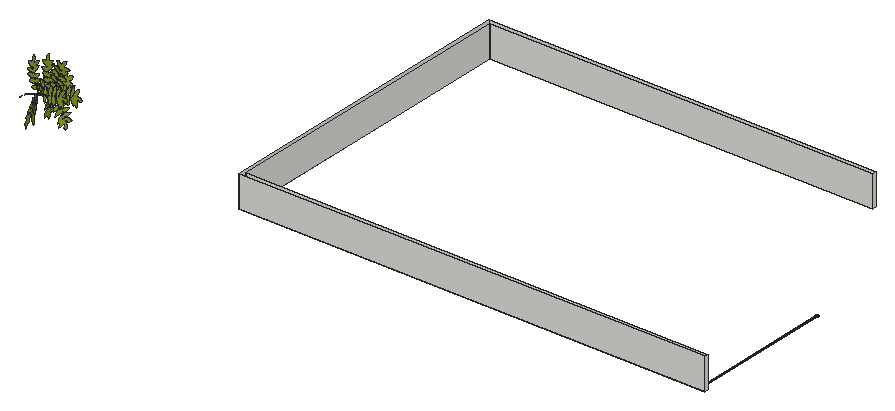
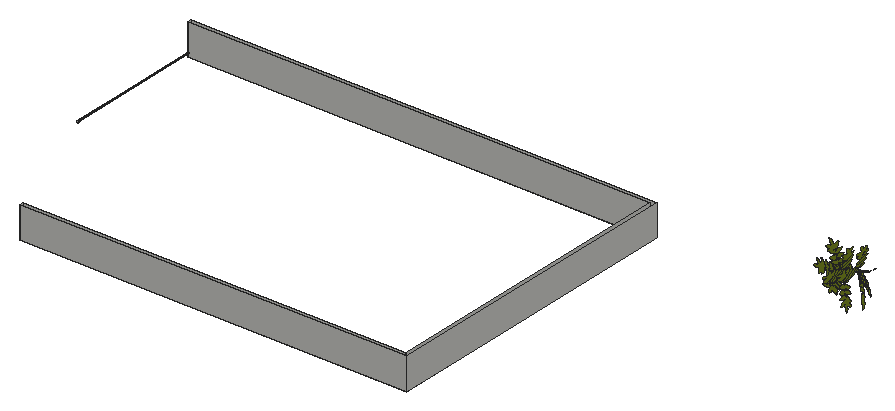
# SketchUp Ruby script. Lengths in inches.
U = 1.inch
M = Sketchup.active_model
def pt(a) = Geom::Point3d.new(a.map { |v| v * U })
def face(e, loops, mat)
  f = e.add_face(loops[0].map { |a| pt(a) })
  loops[1..].each { |l| e.add_face(l.map { |a| pt(a) }).erase! }
  f.material = f.back_material = mat if mat
  f
end
# faces: each face lists its corners as indices into pts; further lists are holes
def faces(e, pts, list, mat = nil) = list.each { |f| face(e, (f[0].is_a?(Array) ? f : [f]).map { |l| l.map { |i| pts[i] } }, mat) }
# xy, xz, yz: faces in a plane at the given z, y or x. An outline is a flat list of corners, or four numbers for a rectangle; further outlines are holes
def ring(l) = l.size == 4 ? [[l[0], l[1]], [l[2], l[1]], [l[2], l[3]], [l[0], l[3]]] : l.each_slice(2).to_a
def flat(e, list, mat, &to3) = list.each { |f| face(e, (f[0].is_a?(Array) ? f : [f]).map { |l| ring(l).map { |u, v| to3.(u, v) } }, mat) }
def xy(e, z, list, mat = nil) = flat(e, list, mat) { |x, y| [x, y, z] }
def xz(e, y, list, mat = nil) = flat(e, list, mat) { |x, z| [x, y, z] }
def yz(e, x, list, mat = nil) = flat(e, list, mat) { |y, z| [x, y, z] }
def lines(e, pts, list) = list.each { |a, b| e.add_line(pt(pts[a]), pt(pts[b])) }
# prism: a flat outline (further loops are holes) pulled along v
def prism(e, loops, v, mat = nil)
  f = face(e, loops, mat); d = Geom::Vector3d.new(v.map { |x| x * U })
  f.pushpull(f.normal.samedirection?(d) ? d.length : -d.length)
end
def box(e, o, s, mat = nil) = prism(e, [[o, [o[0] + s[0], o[1], o[2]], [o[0] + s[0], o[1] + s[1], o[2]], [o[0], o[1] + s[1], o[2]]]], [0, 0, s[2]], mat)
def at(x, y, z, deg = 0) = Geom::Transformation.translation(pt([x, y, z])) * Geom::Transformation.rotation(ORIGIN, Z_AXIS, deg.degrees)
def axes(o, x, y, z) = Geom::Transformation.new([*x, 0, *y, 0, *z, 0, *pt(o).to_a, 1])
def part(name) = M.definitions.add(name)
# library, detail: a bought-in or finely detailed component or shape, given as its bounding box
def library(name, o, s) = part(name).tap { |d| box(d.entities, o, s) }
def detail(e, o, s) = box(e.add_group.entities, o, s)
def put(e, d, t, mat = nil) = e.add_instance(d, t).tap { |i| i.material = mat if mat }
def group(e, t, mat = nil) = e.add_group.tap { |g| g.transformation = t; g.material = mat if mat }.entities
root = M.entities
M.materials.add("3D66_SU_1574822641685_001").color = [135, 150, 36]
M.materials.add("3D66_SU_1574822641883_002").color = [178, 165, 164]
M.materials.add("[Aluminum]").color = [150, 150, 150]
M.materials["[Aluminum]"].alpha = 0.5
c1 = part("rama-acacia")
p = [[-13.8,1.01,-1.08],[-13.61,0.91,-1.04],[-13.61,0.85,-1.06],[-14.07,0.85,-1.21],[-15.17,0.86,-1.58],[-15.95,0.92,-1.83],
  [-16.01,1,-1.83],[-16.01,1.17,-1.78],[-16.07,1.93,-1.6],[-16.4,2.73,-1.5],[-16.65,3.06,-1.5],[-17.13,4.01,-1.41],
  [-17.78,4.7,-1.44],[-18.28,5.07,-1.51],[-18.57,5.18,-1.58],[-18.91,5.47,-1.62],[-19.07,5.48,-1.67],[-19.35,5.61,-1.73],
  [-19.51,5.64,-1.78],[-19.38,5.57,-1.75],[-19.33,5.5,-1.75],[-19.31,5.23,-1.82],[-19.38,5.08,-1.89],[-19.41,4.84,-1.96],
  [-19.36,4.59,-2.01],[-19.43,4.55,-2.04],[-19.36,4.15,-2.125],[-19.21,3.7,-2.19],[-18.875,3.1,-2.24],[-18.61,2.78,-2.24],
  [-17.83,2.19,-2.13],[-17.4375,1.85,-2.09],[-17.04,1.49,-2.05],[-16.61,1.24,-1.97],[-16.17,1.0625,-1.87],[-16.06,0.95,-1.86],
  [-16.06,0.91,-1.87],[-16.32,0.9,-1.96],[-16.7,0.88,-2.1],[-17.05,0.91,-2.21],[-17.61,1.15,-2.33],[-18.06,1.29,-2.45],
  [-18.88,1.53,-2.67],[-20.25,1.46,-3.15],[-20.59,1.49,-3.26],[-20.79,1.37,-3.36],[-21.08,1.2,-3.5],[-21.28,1.22,-3.5625],
  [-21.48,0.94,-3.71],[-21.79,0.5,-3.93],[-22.02,0.17,-4.1],[-22.11,0.05,-4.16],[-22.21,-0.02,-4.21],[-22.375,-0.05,-4.28],
  [-22.375,-0.07,-4.28],[-22.18,-0.09,-4.22],[-22.11,-0.07,-4.19],[-21.78,-0.1,-4.09],[-21.6,-0.18,-4.05],[-21.52,-0.27,-4.04],
  [-21.33,-0.33,-4],[-20.94,-0.54,-3.92],[-20.6875,-0.63,-3.86],[-20.54,-0.68,-3.82],[-20.42,-0.67,-3.78],[-20.09,-0.46,-3.61],
  [-19.8,-0.24,-3.45],[-19.21,-0.02,-3.19],[-18.48,0.08,-2.92],[-17.72,0.38,-2.58],[-17.4,0.5,-2.4375],[-16.93,0.75,-2.21],
  [-16.78,0.8,-2.15],[-16.1,0.83,-1.91],[-16.0625,0.81,-1.9],[-16.08,0.77,-1.91],[-16.27,0.72,-1.99],[-16.88,0.39,-2.29],
  [-17.1875,0.15,-2.46],[-17.27,0.02,-2.52],[-17.94,-0.52,-2.89],[-17.94,-0.59,-2.91],[-18.08,-0.68,-2.99],[-18.13,-0.86,-3.05],
  [-18.56,-1.55,-3.38],[-18.71,-2.11,-3.58],[-18.79,-2.61,-3.74],[-18.86,-2.84,-3.83],[-18.87,-3.07,-3.89],[-18.84,-3.22,-3.92],
  [-18.8,-3.26,-3.92],[-18.76,-3.47,-3.96],[-18.76,-3.6,-4],[-18.67,-3.8,-4.02],[-18.61,-3.92,-4.04],[-18.58,-4.11,-4.07],
  [-18.53,-4.18,-4.08],[-18.58,-4.35,-4.14],[-18.65,-4.43,-4.18],[-18.72,-4.51,-4.23],[-18.8125,-4.51,-4.26],[-18.8125,-4.53,-4.26],
  [-18.72,-4.54,-4.24],[-18.66,-4.49,-4.21],[-18.58,-4.43,-4.16],[-18.35,-4.23,-4.03],[-18.32,-4.17,-4],[-18.22,-4.125,-3.95],
  [-18.1,-4,-3.88],[-17.79,-3.72,-3.7],[-17.68,-3.51,-3.61],[-17.32,-3.13,-3.38],[-17.24,-2.94,-3.31],[-16.78,-2.12,-2.93],
  [-16.48,-1.78,-2.73],[-16.3,-1.28,-2.54],[-16.05,-0.75,-2.3125],[-15.89,-0.2,-2.11],[-15.89,0.39,-1.95],[-15.96,0.79,-1.87],
  [-15.91,0.82,-1.84],[-15.27,0.8,-1.63],[-14.18,0.76,-1.27],[-13.78,0.73,-1.15],[-13.78,0.67,-1.16],[-14.23,0.54,-1.35],
  [-14.65,0.33,-1.55],[-14.97,0.02,-1.74],[-15.25,-0.36,-1.9375],[-15.57,-0.72,-2.14],[-15.96,-1.64,-2.52],[-16.2,-2.51,-2.84],
  [-16.2,-3.12,-3],[-16.14,-3.41,-3.06],[-16.1,-3.75,-3.14],[-16.1,-4.09,-3.23],[-16.2,-4.25,-3.3],[-16.2,-4.28,-3.3125],
  [-16.08,-4.19,-3.24],[-15.98,-4.08,-3.18],[-15.96,-3.94,-3.14],[-15.96,-3.8125,-3.1],[-15.9,-3.72,-3.06],[-15.68,-3.55,-2.9375],
  [-15.51,-3.49,-2.86],[-15.3,-3.33,-2.75],[-15.23,-3.17,-2.68],[-15.01,-3.03,-2.57],[-14.875,-2.83,-2.47],[-14.6,-2.59,-2.3125],
  [-14.4,-2.27,-2.16],[-14.12,-1.6,-1.89],[-13.91,-1.1,-1.68],[-13.67,-0.83,-1.53],[-13.53,-0.45,-1.38],[-13.53,0.67,-1.08],
  [-13.53,0.69,-1.07],[-13.38,0.86,-0.98],[-13.38,0.92,-0.96],[-13.32,1.03,-0.91],[-13.32,1.35,-0.82],[-13.28,1.49,-0.77],
  [-13.28,1.99,-0.64],[-13.44,2.67,-0.51],[-13.72,3.31,-0.43],[-13.93,3.71,-0.4],[-14.1,4.39,-0.27],[-14.5625,5.06,-0.25],
  [-14.89,5.62,-0.21],[-15.33,6.1,-0.23],[-15.65,6.8,-0.15],[-15.79,6.89,-0.18],[-15.61,6.52,-0.22],[-15.51,6.32,-0.24],
  [-15.45,6.28,-0.23],[-15.52,6,-0.32],[-15.63,5.6875,-0.45],[-15.77,4.97,-0.68],[-15.7,4.25,-0.85],[-15.46,3,-1.11],
  [-15,2.03,-1.21],[-14.3,1.29,-1.17],[-12.41,6.01,0.65],[-12.44,6.14,0.68],[-12.41,6.29,0.73],[-12.43,6.29,0.73],
  [-12.44,6.26,0.72],[-12.47,6.15,0.68],[-12.49,6.07,0.66],[-12.57,5.75,0.55],[-12.67,5.36,0.43],[-12.79,4.875,0.28],
  [-12.83,4.52,0.18],[-12.83,3.99,0.04],[-12.73,3.11,-0.18],[-12.58,2.52,-0.3125],[-12.3,1.97,-0.41],[-11.88,1.51,-0.46],
  [-11.37,1.0625,-0.48],[-10.75,0.75,-0.45],[-10.75,0.68,-0.47],[-12.55,0.7,-0.79],[-13.21,0.79,-0.89],[-13.2,0.67,-0.92],
  [-12.56,0.62,-0.82],[-11.15,0.56,-0.58],[-10.79,0.54,-0.52],[-10.72,0.52,-0.51],[-10.72,0.5,-0.52],[-10.87,0.47,-0.55],
  [-11.14,0.41,-0.62],[-11.39,0.27,-0.7],[-11.625,-0.01,-0.82],[-11.8,-0.43,-0.96],[-11.83,-0.57,-1],[-12.02,-1.08,-1.17],
  [-12.1,-1.39,-1.27],[-12.17,-1.95,-1.4375],[-12.17,-2.77,-1.65],[-12.09,-3.59,-1.86],[-11.86,-4.26,-2],[-11.8125,-4.4,-2.03],
  [-11.84,-4.49,-2.05],[-11.91,-4.6,-2.1],[-11.97,-4.65,-2.12],[-11.98,-4.67,-2.13],[-11.92,-4.65,-2.11],[-11.84,-4.59,-2.08],
  [-11.77,-4.52,-2.05],[-11.74,-4.47,-2.03],[-11.37,-4.3125,-1.92],[-10.95,-4.0625,-1.78],[-10.82,-3.89,-1.71],[-10.64,-3.57,-1.59],
  [-10.41,-3.05,-1.41],[-10.27,-2.73,-1.3],[-10.07,-1.88,-1.03],[-10.15,-0.71,-0.73],[-10.31,-0.1,-0.6],[-10.5,0.4,-0.5],
  [-10.5,0.48,-0.48],[-10.44,0.53,-0.45],[-10.39,0.64,-0.42],[-10.52,0.73,-0.42],[-10.44,0.93,-0.35],[-10.44,1.2,-0.28],
  [-10.32,1.47,-0.18],[-10.48,2.6875,0.12],[-10.43,2.96,0.2],[-10.75,3.87,0.38],[-11.26,4.93,0.57],[-11.8,5.54,0.64],
  [-12.37,5.93,0.64],[-7.78,0.19,-0.06],[-7.78,0.25,-0.04],[-7.75,0.39,0],[-7.89,0.4,-0.02],[-7.96,0.46,-0.02],
  [-7.96,0.49,-0.01],[-7.76,0.62,0.06],[-7.53,0.99,0.2],[-7.31,1.78,0.45],[-7.31,2.74,0.71],[-7.63,3.6875,0.9],
  [-8.02,4.57,1.07],[-8.66,5.23,1.13],[-8.83,5.4,1.14],[-8.92,5.54,1.16],[-9.1,5.64,1.16],[-9.08,5.6,1.15],
  [-9.02,5.56,1.15],[-8.94,5.46,1.14],[-8.9,5.37,1.12],[-8.9375,5.25,1.08],[-9.14,4.92,0.96],[-9.31,4.5625,0.83],
  [-9.39,3.73,0.6],[-9.44,2.76,0.32],[-9.23,1.59,0.05],[-8.82,0.9,-0.06],[-8.36,0.59,-0.0625],[-8.14,0.51,-0.04],
  [-8.05,0.48,-0.03],[-8.05,0.46,-0.04],[-8.12,0.43,-0.06],[-10.1,0.49,-0.4],[-8.22,0.3125,-0.11],[-8.22,0.25,-0.125],
  [-8.53,0.13,-0.21],[-8.8,-0.16,-0.34],[-8.96,-0.61,-0.49],[-8.96,-0.87,-0.56],[-9.16,-1.42,-0.74],[-9.13,-1.77,-0.83],
  [-9.09,-1.83,-0.84],[-9.125,-1.92,-0.87],[-9.125,-2.13,-0.93],[-9.08,-2.23,-0.95],[-9.15,-2.39,-1],[-9.11,-2.67,-1.07],
  [-9.03,-2.86,-1.11],[-9.07,-3.03,-1.16],[-8.97,-3.23,-1.19],[-8.93,-3.44,-1.24],[-8.93,-3.71,-1.32],[-8.79,-4.05,-1.38],
  [-8.7,-4.25,-1.42],[-8.7,-4.39,-1.46],[-8.76,-4.53,-1.5],[-8.77,-4.65,-1.54],[-8.64,-4.55,-1.49],[-8.27,-4.22,-1.33],
  [-8.1875,-4.06,-1.27],[-8.07,-3.98,-1.23],[-7.98,-3.79,-1.17],[-7.79,-3.59,-1.08],[-7.64,-3.3,-0.97],[-7.64,-3.25,-0.96],
  [-7.59,-3.21,-0.9375],[-7.52,-2.93,-0.85],[-7.52,-2.85,-0.83],[-7.47,-2.81,-0.81],[-7.3,-2.09,-0.59],[-7.32,-2.01,-0.57],
  [-7.27,-1.95,-0.54],[-7.1875,-1.57,-0.42],[-7.17,-1.46,-0.39],[-7.17,-1.16,-0.3125],[-7.23,-0.61,-0.17],[-7.49,-0.15,-0.1],
  [-13.39,-0.07,-1.23],[-13.39,0.25,-1.14],[-13.49,0.5625,-1.09],[-4.5625,0.33,0.09],[-4.22,0.49,0.13],[-4,0.7,0.1875],
  [-3.86,0.99,0.26],[-3.77,1.41,0.38],[-3.7,1.73,0.46],[-3.77,1.99,0.53],[-3.85,2.17,0.58],[-3.88,2.57,0.6875],
  [-3.98,2.9,0.78],[-4.0625,2.97,0.8],[-4.1,3.14,0.84],[-4.1875,3.25,0.87],[-4.27,3.55,0.95],[-4.31,3.71,0.99],
  [-4.42,3.9,1.04],[-4.625,4.2,1.125],[-4.72,4.39,1.18],[-4.89,4.57,1.23],[-4.98,4.73,1.27],[-5,4.72,1.26],
  [-5.01,4.51,1.21],[-4.96,4.32,1.16],[-4.97,4.27,1.14],[-5.14,3.78,1.01],[-5.3,3.39,0.91],[-5.44,2.76,0.74],
  [-5.5,2.09,0.56],[-5.57,1.78,0.48],[-5.57,1.42,0.38],[-5.57,1.09,0.29],[-5.47,0.72,0.19],[-5.22,0.44,0.12],
  [-4.93,0.27,0.07],[-4.76,0.22,0.06],[-4.76,0.18,0.05],[-4.83,0.16,0.04],[-5.26,0,0],[-5.34,-0.04,-0.01],
  [-5.47,-0.22,-0.06],[-5.51,-0.6,-0.16],[-5.42,-1.09,-0.29],[-5.28,-1.49,-0.4],[-5.21,-1.87,-0.5],[-5.11,-2.15,-0.57],
  [-5.08,-2.34,-0.63],[-5.01,-2.47,-0.66],[-4.96,-2.69,-0.72],[-4.86,-2.9375,-0.79],[-4.84,-3.07,-0.82],[-4.77,-3.18,-0.85],
  [-4.74,-3.43,-0.92],[-4.7,-3.71,-0.99],[-4.62,-3.89,-1.04],[-4.58,-3.98,-1.07],[-4.58,-3.83,-1.03],[-4.51,-3.67,-0.98],
  [-4.3,-3.32,-0.89],[-4.16,-3.09,-0.83],[-4.16,-2.98,-0.8],[-4.11,-2.92,-0.78],[-4.02,-2.8,-0.75],[-3.95,-2.59,-0.69],
  [-3.95,-2.33,-0.625],[-3.86,-2.26,-0.6],[-3.86,-2.02,-0.54],[-3.86,-1.44,-0.39],[-3.94,-1.22,-0.33],[-3.94,-1.08,-0.29],
  [-4,-0.96,-0.26],[-4,-0.87,-0.23],[-4.0625,-0.8125,-0.22],[-4.16,-0.54,-0.14],[-4.39,-0.24,-0.06],[-4.61,-0.08,-0.02],
  [-4.77,-0.03,-0.01],[-4.77,-0.01,0],[-4.65,-0.01,0],[-4.61,0.19,0.05],[-4.66,0.23,0.0625],[-4.63,0.29,0.08],
  [-4.07,0.17,0.04],[0,-0.24,-0.06],[0,0,0],[-0.5,0.04,0.01],[-1.58,0.08,0.02]]
faces(c1.entities,p,[[0,1,2,3,4,5,6,7,8,9,10,11,12,13,14,15,16,17,18,19,20,21,22,23,24,25,26,27,28,29,30,31,32,33,34,35,36,37,38,39,40,41,42,43,44,45,46,47,48,49,50,51,52,53,54,55,56,57,58,59,60,61,62,63,64,65,66,67,68,69,70,71,72,73,74,75,76,77,78,79,80,81,82,83,84,85,86,87,88,89,90,91,92,93,94,95,96,97,98,99,100,101,102,103,104,105,106,107,108,109,110,111,112,113,114,115,116,117,118,119,120,121,122,123,124,125,126,127,128,129,130,131,132,133,134,135,136,137,138,139,140,141,142,143,144,145,146,147,148,149,150,151,152,153,154,155,156,157,158,159,160,161,162,163,164,165,166,167,168,169,170,171,172,173,174,175,176,177,178,179,180,181],[182,183,184,185,186,187,188,189,190,191,192,193,194,195,196,197,198,199,200,201,202,203,204,205,206,207,208,209,210,211,212,213,214,215,216,217,218,219,220,221,222,223,224,225,226,227,228,229,230,231,232,233,234,235,236,237,238,239,240,241,242,243,244,245,246,247,248,249,250,251,252],[253,254,255,256,257,258,259,260,261,262,263,264,265,266,267,268,269,270,271,272,273,274,275,276,277,278,279,280,281,282,283,284,242,241,285,286,287,288,289,290,291,292,293,294,295,296,297,298,299,300,301,302,303,304,305,306,307,308,309,310,311,312,313,314,315,316,317,318,319,320,321,322,323,324,325,326,327,328,329],[154,330,331,332,155],[333,334,335,336,337,338,339,340,341,342,343,344,345,346,347,348,349,350,351,352,353,354,355,356,357,358,359,360,361,362,363,364,365,366,367,368,369,370,371,372,373,374,375,376,377,378,379,380,381,382,383,384,385,386,387,388,389,390,391,392,393,394,395,396,397,398,399,400,401,402,403,404,405,406,407,408,409,410,411,412,413],[156,203,157],[202,157,203],[414,411,410,415,416,417,418],
  [254,370,255],[369,255,370]],"3D66_SU_1574822641685_001")
c2 = part("ramas")
put(c2.entities,c1,axes([0.11,0.06,-0.22],[-0.42655,-0.79206,-0.43668],[0.22445,0.37501,-0.89944],[0.87617,-0.48167,0.01782]))
put(c2.entities,c1,axes([0.14,0.21,0.02],[0.24321,-0.08852,-0.96593],[0.34202,0.93969,0],[0.90767,-0.33037,0.25882]))
put(c2.entities,c1,at(0,0.24,0.06))
put(c2.entities,c1,axes([0.11,0.45,0.57],[-0.42655,0.68302,0.5929],[0.22445,-0.55509,0.80093],[0.87617,0.47472,0.08347]))
put(c2.entities,c1,axes([0.11,0.73,0.01],[-0.42655,0.88928,-0.16503],[0.22445,0.28083,0.93314],[0.87617,0.36099,-0.31939]))
c3 = part("rama principal")
put(c3.entities,c1,axes([-20.25,-0.15,12.84],[0.38818,-0.89018,-0.23852],[0.89018,0.42916,-0.15296],[0.23852,-0.15296,0.95902]))
put(c3.entities,c1,at(-20.48,0,12.88))
put(c3.entities,c1,axes([-20.6875,-0.1,12.85],[0.57358,0.79124,0.21201],[-0.79124,0.60214,-0.10661],[-0.21201,-0.10661,0.97144]))
put(c3.entities,c1,axes([-20.375,-0.01,13.02],[-0.37792,0.77975,-0.49916],[-0.65887,0.15226,0.73669],[0.65043,0.60729,0.45621]))
put(c3.entities,c1,axes([-20.34,-0.04,12.83],[0.24321,-0.08852,-0.96593],[0.34202,0.93969,0],[0.90767,-0.33037,0.25882]))
put(c3.entities,c1,axes([-20.375,-0.18,12.6],[-0.42655,-0.79206,-0.43668],[0.22445,0.37501,-0.89944],[0.87617,-0.48167,0.01782]))
put(c3.entities,c2,at(-11.43,0,7.77))
g1 = group(c3.entities,at(0,0.2,0),"3D66_SU_1574822641883_002")
xz(g1,0.1,[[-0.15,-0.08,-3.26,5.59,-11.5,7.61,-18.23,12.71,-20.48,12.71,-20.48,13.05,-18.11,13.05,-11.35,7.92,-3.03,5.89,0.15,0.08]])
yz(g1,-20.48,[[0.1,12.71,-0.2,12.88,0.1,13.05]])
p = [[-0.15,0.1,-0.08],[0,-0.2,0],[-3.15,-0.2,5.74],[-3.26,0.1,5.59],[0.15,0.1,0.08],[-3.03,0.1,5.89],
  [-11.43,-0.2,7.77],[-11.5,0.1,7.61],[-11.35,0.1,7.92],[-18.17,-0.2,12.88],[-18.23,0.1,12.71],[-18.11,0.1,13.05],
  [-20.48,-0.2,12.88],[-20.48,0.1,12.71],[-20.48,0.1,13.05]]
faces(g1,p,[[0,1,2,3],[0,4,1],[1,4,5,2],[3,2,6,7],[2,5,8,6],[7,6,9,10],[6,8,11,9],[10,9,12,13],
  [9,11,14,12]])
xy(root,121.94,[[334.375,113.59,334.375,473.59,779.5,473.59,779.5,468.87,338.3125,468.87,338.3125,117.53,871.06,117.53,871.06,113.59]])
xy(root,125.65,[[869.01,117.53,869.09,278.08]],"[Aluminum]")
xy(root,127.64,[[869.09,117.53,869.17,278.08]],"[Aluminum]")
xz(root,113.59,[[334.375,121.94,871.06,158.24]])
xz(root,117.53,[[[338.3125,121.94,871.06,158.24],[869.01,129.71,869.09,129.71,869.27,129.72,869.52,129.8,869.74,129.94,869.91,130.14,870.03,130.37,870.09,130.62,870.07,130.88,869.99,131.13,869.85,131.35,869.66,131.53,869.43,131.65,869.17,131.7,869.09,131.7,868.91,131.6875,868.66,131.61,868.44,131.47,868.27,131.27,868.15,131.04,868.09,130.79,868.11,130.53,868.19,130.28,868.33,130.06,868.52,129.88,868.75,129.76],[869.01,125.65,869.09,125.65,869.27,125.66,869.52,125.74,869.74,125.88,869.91,126.07,870.03,126.3,870.09,126.56,870.07,126.82,869.99,127.07,869.85,127.29,869.66,127.46,869.43,127.58,869.17,127.64,869.09,127.64,868.91,127.625,868.66,127.55,868.44,127.41,868.27,127.21,868.15,126.98,868.09,126.73,868.11,126.46,868.19,126.22,868.33,126,868.52,125.82,868.75,125.7],[869.01,133.65,869.09,133.65,869.27,133.66,869.52,133.74,869.74,133.88,869.91,134.08,870.03,134.31,870.09,134.5625,870.07,134.82,869.99,135.07,869.85,135.29,869.66,135.47,869.43,135.59,869.17,135.64,869.09,135.64,868.91,135.63,868.66,135.55,868.44,135.41,868.27,135.21,868.15,134.98,868.09,134.73,868.11,134.47,868.19,134.22,868.33,134,868.52,133.82,868.75,133.7],[869.01,137.55,869.09,137.55,869.27,137.5625,869.52,137.64,869.74,137.78,869.91,137.98,870.03,138.21,870.09,138.46,870.07,138.72,869.99,138.97,869.85,139.19,869.66,139.37,869.43,139.49,869.17,139.54,869.09,139.54,868.91,139.53,868.66,139.45,868.44,139.31,868.27,139.11,868.15,138.88,868.09,138.63,868.11,138.37,868.19,138.12,868.33,137.9,868.52,137.72,868.75,137.6],[869.01,141.49,869.09,141.49,869.27,141.5,869.52,141.58,869.74,141.72,869.91,141.92,870.03,142.15,870.09,142.4,870.07,142.66,869.99,142.91,869.85,143.13,869.66,143.31,869.43,143.43,869.17,143.48,869.09,143.48,868.91,143.47,868.66,143.39,868.44,143.25,868.27,143.05,868.15,142.82,868.09,142.57,868.11,142.31,868.19,142.06,868.33,141.84,868.52,141.66,868.75,141.54],[869.01,145.43,869.09,145.43,869.27,145.44,869.52,145.52,869.74,145.66,869.91,145.86,870.03,146.09,870.09,146.34,870.07,146.61,869.99,146.85,869.85,147.07,869.66,147.25,869.43,147.37,869.17,147.42,869.09,147.42,868.91,147.41,868.66,147.33,868.44,147.19,868.27,147,868.15,146.77,868.09,146.51,868.11,146.25,868.19,146,868.33,145.78,868.52,145.61,868.75,145.49],[869.01,149.37,869.09,149.37,869.27,149.38,869.52,149.46,869.74,149.6,869.91,149.8,870.03,150.03,870.09,150.28,870.07,150.54,869.99,150.79,869.85,151.01,869.66,151.1875,869.43,151.31,869.17,151.36,869.09,151.36,868.91,151.35,868.66,151.27,868.44,151.13,868.27,150.93,868.15,150.7,868.09,150.45,868.11,150.1875,868.19,149.9375,868.33,149.72,868.52,149.54,868.75,149.42],[869.09,153.3,869.35,153.34,869.59,153.4375,869.8,153.6,869.96,153.8,870.06,154.05,870.09,154.3,870.06,154.5625,869.96,154.8,869.8,155.01,869.59,155.17,869.35,155.27,869.09,155.3,868.83,155.27,868.59,155.17,868.38,155.01,868.22,154.8,868.125,154.5625,868.09,154.3,868.125,154.05,868.22,153.8,868.38,153.6,868.59,153.4375,868.83,153.34]]])
xz(root,278.08,[[869.01,125.65,868.75,125.7,868.52,125.82,868.33,126,868.19,126.22,868.11,126.46,868.09,126.73,868.15,126.98,868.27,127.21,868.44,127.41,868.66,127.55,868.91,127.625,869.09,127.64,869.17,127.64,869.43,127.58,869.66,127.46,869.85,127.29,869.99,127.07,870.07,126.82,870.09,126.56,870.03,126.3,869.91,126.07,869.74,125.88,869.52,125.74,869.27,125.66,869.09,125.65]])
xz(root,468.87,[[338.3125,121.94,779.5,158.24]])
xz(root,473.59,[[334.375,121.94,779.5,158.24]])
yz(root,334.375,[[113.59,121.94,473.59,158.24]])
yz(root,338.3125,[[117.53,121.94,468.87,158.24]])
yz(root,779.5,[[468.87,121.94,473.59,158.24]])
yz(root,871.06,[[113.59,121.94,117.53,158.24]])
p = [[869.01,117.53,125.65],[868.75,117.53,125.7],[868.75,278.08,125.7],[869.01,278.08,125.65],[869.27,117.53,125.66],[869.09,117.53,125.65],
  [869.09,278.08,125.65],[869.27,278.08,125.66],[868.52,117.53,125.82],[868.52,278.08,125.82],[869.52,117.53,125.74],[869.52,278.08,125.74],
  [869.74,117.53,125.88],[869.74,278.08,125.88],[868.33,117.53,126],[868.33,278.08,126],[869.91,117.53,126.07],[869.91,278.08,126.07],
  [868.19,117.53,126.22],[868.19,278.08,126.22],[870.03,117.53,126.3],[870.03,278.08,126.3],[868.11,117.53,126.46],[868.11,278.08,126.46],
  [870.09,117.53,126.56],[870.09,278.08,126.56],[868.09,117.53,126.73],[868.09,278.08,126.73],[870.07,117.53,126.82],[870.07,278.08,126.82],
  [868.15,117.53,126.98],[868.15,278.08,126.98],[869.99,117.53,127.07],[869.99,278.08,127.07],[868.27,117.53,127.21],[868.27,278.08,127.21],
  [869.85,117.53,127.29],[869.85,278.08,127.29],[868.44,117.53,127.41],[868.44,278.08,127.41],[869.66,117.53,127.46],[869.66,278.08,127.46],
  [868.66,117.53,127.55],[868.66,278.08,127.55],[868.91,117.53,127.625],[868.91,278.08,127.625],[869.43,117.53,127.58],[869.43,278.08,127.58],
  [869.09,117.53,127.64],[869.09,278.08,127.64],[869.17,117.53,127.64],[869.17,278.08,127.64],[338.3125,468.87,158.24],[338.3125,468.87,121.94]]
faces(root,p,[[0,1,2,3],[4,5,6,7],[1,8,9,2],[10,4,7,11],[12,10,11,13],[8,14,15,9],[16,12,13,17],[14,18,19,15],
  [20,16,17,21],[18,22,23,19],[24,20,21,25],[22,26,27,23],[28,24,25,29],[26,30,31,27],[32,28,29,33],[30,34,35,31],
  [36,32,33,37],[34,38,39,35],[40,36,37,41],[38,42,43,39],[42,44,45,43],[46,40,41,47],[44,48,49,45],[50,46,47,51]],"[Aluminum]")
lines(root,p,[[52,53]])
put(root,c3,axes([98.67,92.73,163.47],[-1.22279,-0.43771,0],[0,0,1.6799],[-0.47,1.13878,0]))
